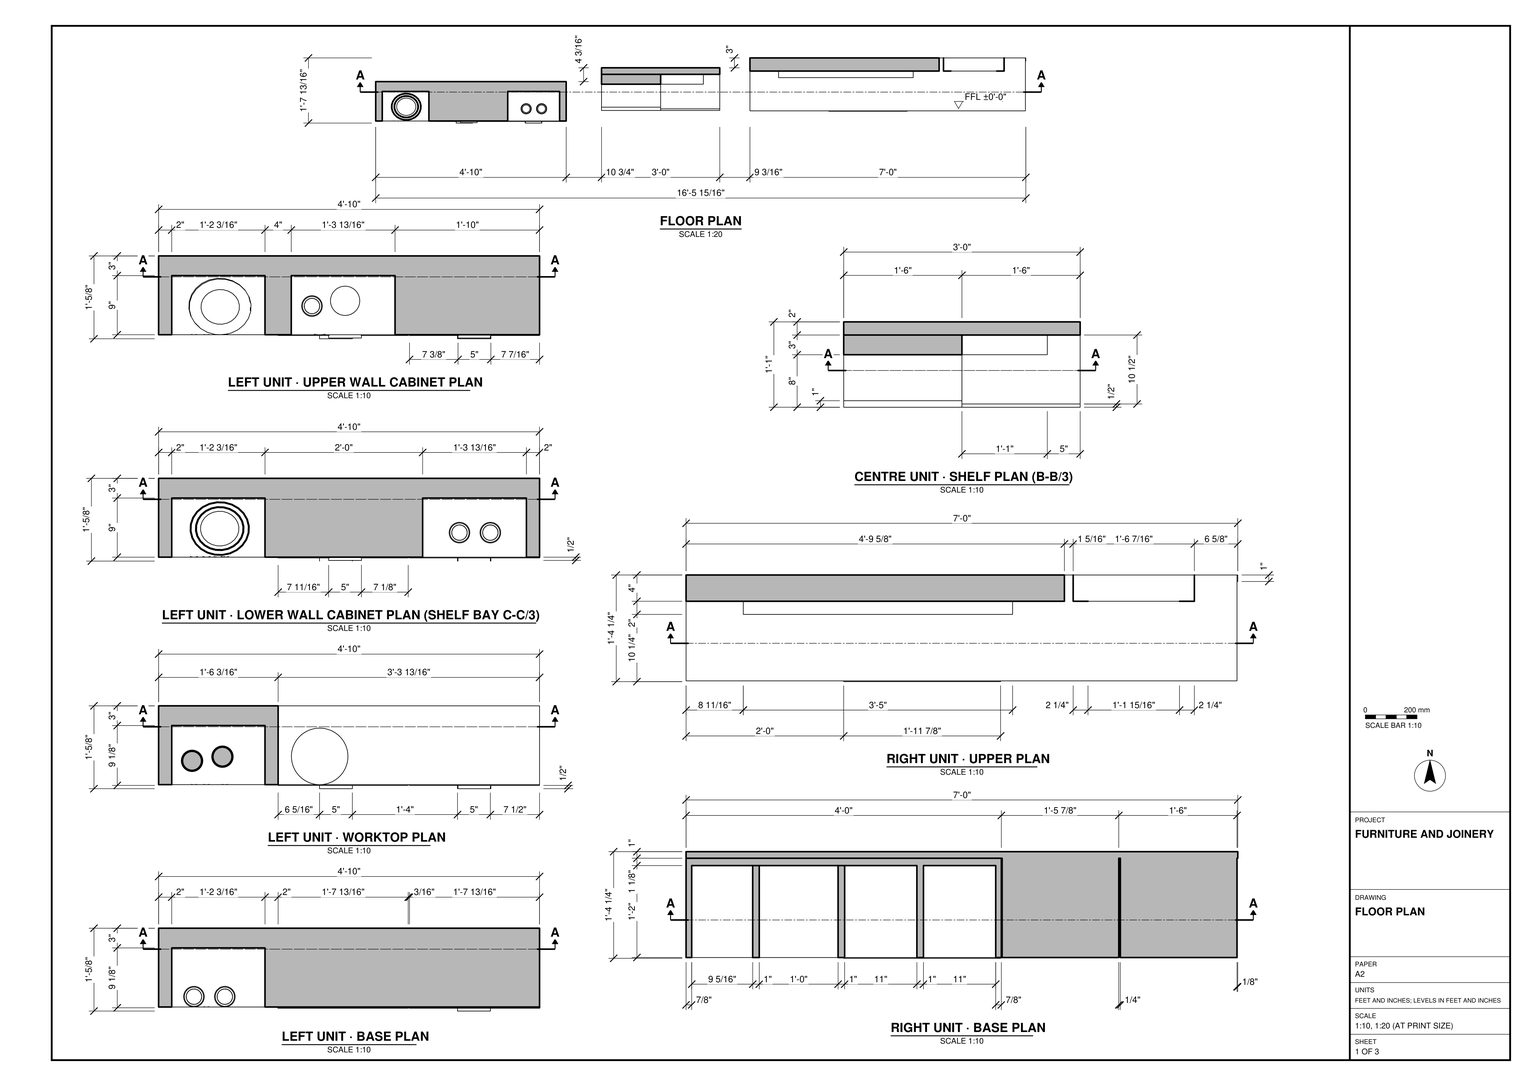
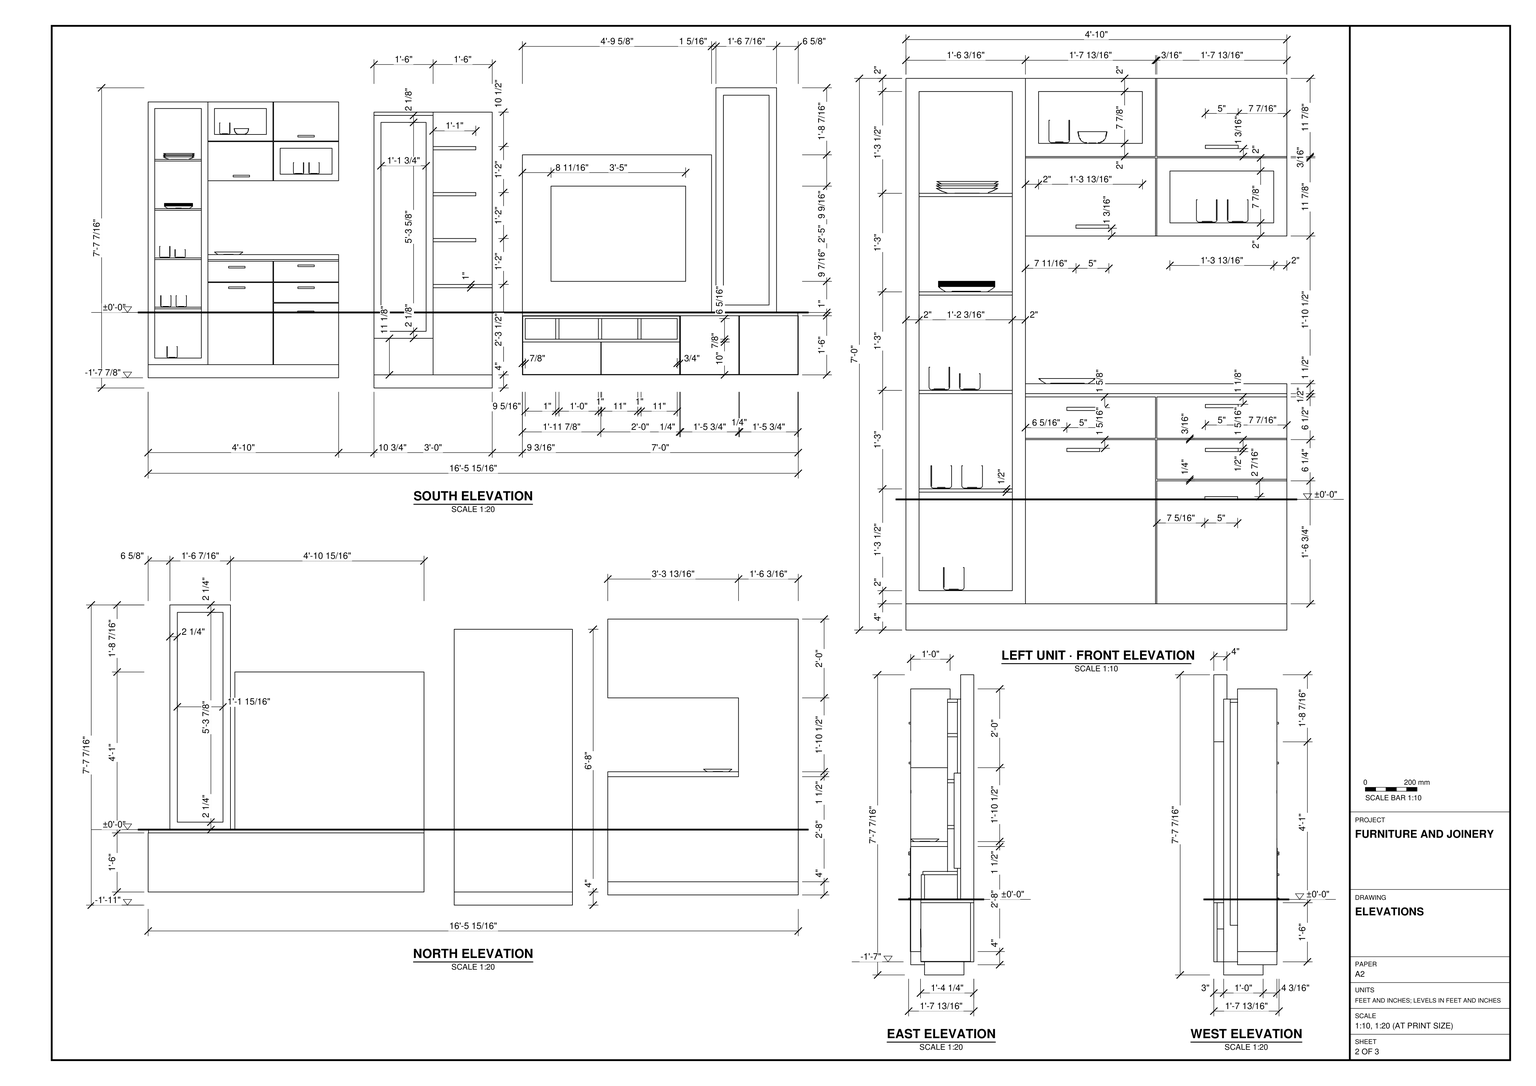
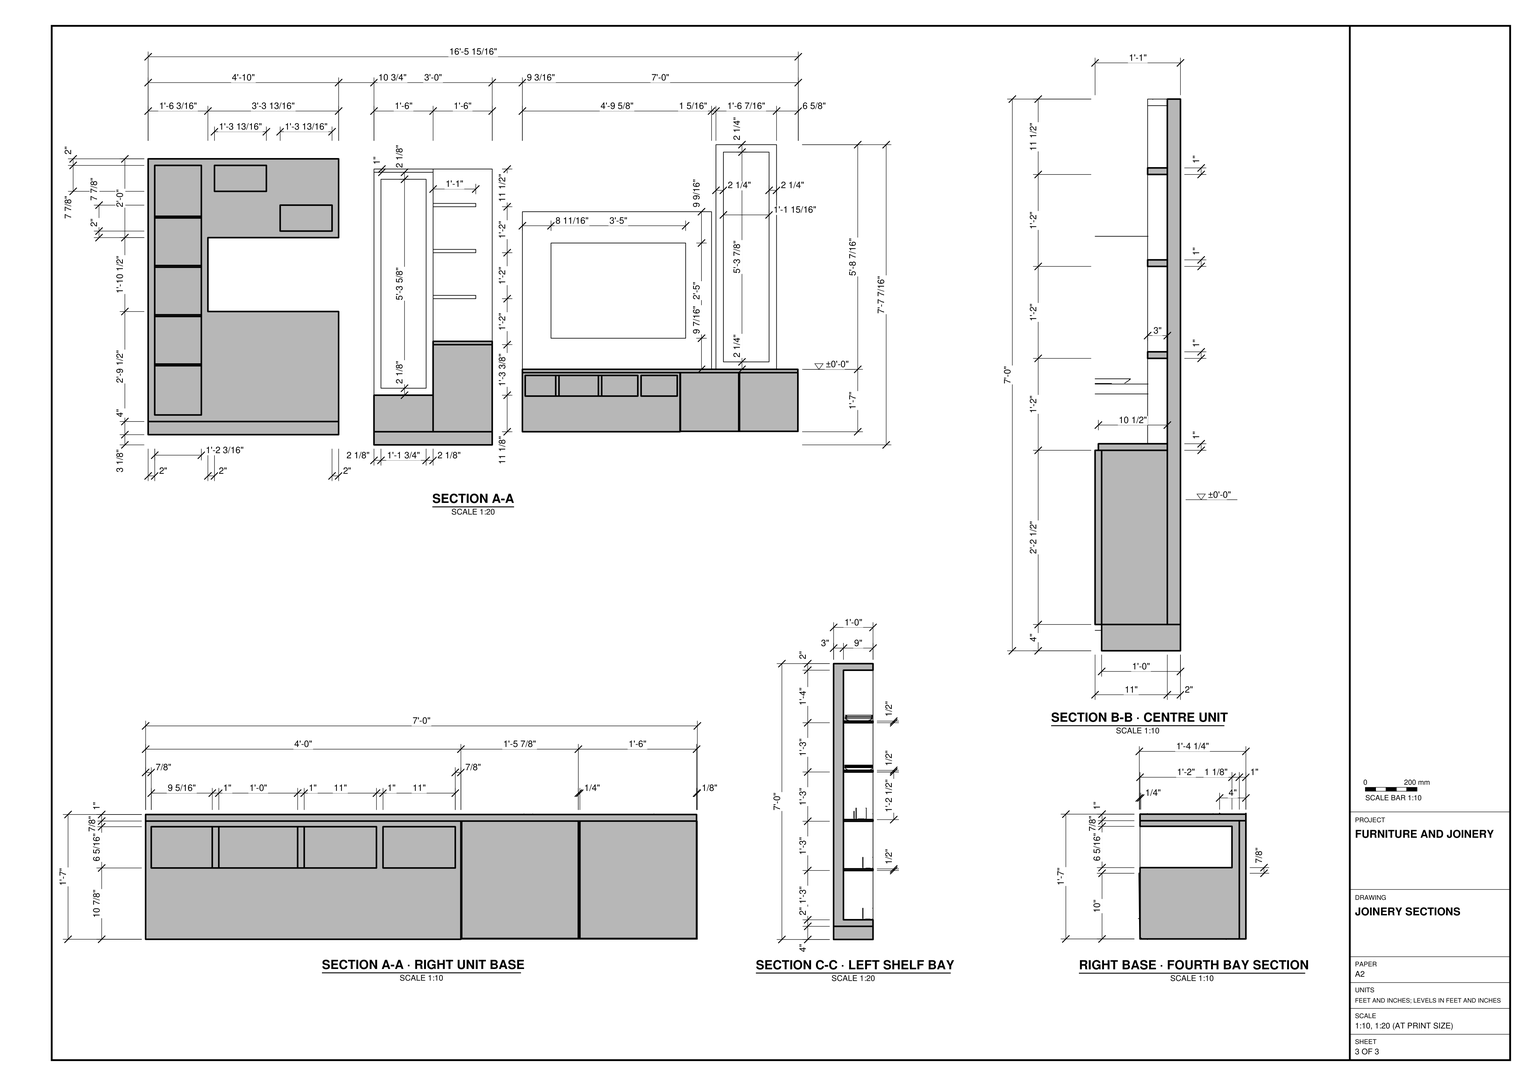
Build the joinery assembly in SketchUp from task_files/diagram_01.pdf. Work in feet and inches, with the finished-floor reference at ±0'-0". The assembly measures 16'-5 15/16" across, 1'-7 13/16" in overall depth and 7'-7 7/16" in overall height. Use the floor plan to set the gaps and front-to-back offsets between the units. Use section A-A to set their bases and tops relative to the reference level; the bases do not all sit at the same height.

On the left, build a full-height open shelf bay beside a worktop with storage below and wall cabinets above. Follow the front elevation for the drawer and cupboard divisions, pulls and open display compartments. In the centre unit, place the tall framed panel on the left and the projecting shelves on the right. On the right unit, build the long low cabinet with a row of shallow open compartments at its left end. Above it, model the wide rectangular panel and the taller, narrower framed panel. Use the detail plans and sections to give the backs, sides, shelves, plinths and fronts their drawn thicknesses and recesses.

Place dishes and cups in the left unit as shown. Decor and loose items may be any suitable library components. Keep each joinery piece in a separate group or component and use components for repeated parts. Save one SketchUp model as output_files/three_part_display_and_storage_unit.skp.

# SketchUp Ruby script. Lengths in inches.
U = 1.inch
M = Sketchup.active_model
def pt(a) = Geom::Point3d.new(a.map { |v| v * U })
def face(e, loops, mat)
  f = e.add_face(loops[0].map { |a| pt(a) })
  loops[1..].each { |l| e.add_face(l.map { |a| pt(a) }).erase! }
  f.material = f.back_material = mat if mat
  f
end
# faces: each face lists its corners as indices into pts; further lists are holes
def faces(e, pts, list, mat = nil) = list.each { |f| face(e, (f[0].is_a?(Array) ? f : [f]).map { |l| l.map { |i| pts[i] } }, mat) }
# xy, xz, yz: faces in a plane at the given z, y or x. An outline is a flat list of corners, or four numbers for a rectangle; further outlines are holes
def ring(l) = l.size == 4 ? [[l[0], l[1]], [l[2], l[1]], [l[2], l[3]], [l[0], l[3]]] : l.each_slice(2).to_a
def flat(e, list, mat, &to3) = list.each { |f| face(e, (f[0].is_a?(Array) ? f : [f]).map { |l| ring(l).map { |u, v| to3.(u, v) } }, mat) }
def xy(e, z, list, mat = nil) = flat(e, list, mat) { |x, y| [x, y, z] }
def xz(e, y, list, mat = nil) = flat(e, list, mat) { |x, z| [x, y, z] }
def yz(e, x, list, mat = nil) = flat(e, list, mat) { |y, z| [x, y, z] }
def lines(e, pts, list) = list.each { |a, b| e.add_line(pt(pts[a]), pt(pts[b])) }
# prism: a flat outline (further loops are holes) pulled along v
def prism(e, loops, v, mat = nil)
  f = face(e, loops, mat); d = Geom::Vector3d.new(v.map { |x| x * U })
  f.pushpull(f.normal.samedirection?(d) ? d.length : -d.length)
end
def box(e, o, s, mat = nil) = prism(e, [[o, [o[0] + s[0], o[1], o[2]], [o[0] + s[0], o[1] + s[1], o[2]], [o[0], o[1] + s[1], o[2]]]], [0, 0, s[2]], mat)
def at(x, y, z, deg = 0) = Geom::Transformation.translation(pt([x, y, z])) * Geom::Transformation.rotation(ORIGIN, Z_AXIS, deg.degrees)
def axes(o, x, y, z) = Geom::Transformation.new([*x, 0, *y, 0, *z, 0, *pt(o).to_a, 1])
def part(name) = M.definitions.add(name)
# library, detail: a bought-in or finely detailed component or shape, given as its bounding box
def library(name, o, s) = part(name).tap { |d| box(d.entities, o, s) }
def detail(e, o, s) = box(e.add_group.entities, o, s)
def put(e, d, t, mat = nil) = e.add_instance(d, t).tap { |i| i.material = mat if mat }
def group(e, t, mat = nil) = e.add_group.tap { |g| g.transformation = t; g.material = mat if mat }.entities
root = M.entities
M.materials.add("[Suede Dark Gray]").color = [85, 85, 85]
M.materials.add("[Wood Cherry Original]").color = [152, 86, 42]
M.materials.add("[Wood Floor Parquet]").color = [145, 89, 39]
M.materials.add("[Wood Veneer 01]").color = [120, 70, 37]
c1 = library("Cup (heat up)",[-27.01,0,-31.5],[48.56,5.94,71.64])
c2 = library("plates",[-46.18,-12,0],[25.68,8.61,38.39])
c3 = library("plates\#1",[10.82,85.4,0],[80.06,80.43,16.52])
c4 = part("Group\#8")
box(c4.entities,[0,0,0],[5,0.5,0.5])
c5 = part("Group\#3")
box(c5.entities,[0,0,0],[14.2,9,0.5])
c6 = part("Group\#4")
put(c6.entities,c5,at(0,0,0))
c7 = part("Group\#26")
g1 = group(c7.entities,at(0,0,0))
box(g1,[0,0,0],[13,1,3])
box(root,[38.2,0.5,8.72],[19.8,0.12,6.31])
box(root,[18.2,0.5,8.72],[19.8,0.12,6.31])
xy(root,-19.58,[[68.77,4.83,86.77,14.83],[86.77,4.83,104.77,14.83],[68.77,14.83,104.77,16.83]])
xy(root,-16.47,[[18.2,0.5,38,0.62],[38.2,0.5,58,0.62]])
xy(root,-8.45,[[68.77,4.83,86.77,11.83],[68.77,11.83,86.77,14.83]])
xy(root,2.25,[[38.2,0.5,58,0.62]])
xy(root,2.49,[[38.2,0.5,58,0.62]])
xy(root,6.94,[[86.77,4.83,104.77,14.83]])
xy(root,8.52,[[18.2,0.5,38,0.62],[38.2,0.5,58,0.62]])
xy(root,60.42,[[68.77,14.83,104.77,16.83]])
xz(root,0.5,[[18.2,-16.47,38,8.52],[38.2,-16.47,58,2.25],[38.2,2.49,58,8.52]],"[Wood Veneer 01]")
xz(root,0.62,[[18.2,-16.47,38,8.52],[38.2,-16.47,58,2.25],[38.2,2.49,58,8.52]])
xz(root,4.83,[[68.77,-19.58,86.77,-8.45]])
xz(root,11.83,[[[68.77,-8.45,86.77,59.42],[70.89,-6.33,84.65,57.3]],[70.89,-6.33,84.65,57.3]])
xz(root,14.83,[[86.77,-19.58,104.77,6.94],[68.77,-8.45,86.77,-8.45,86.77,6.94,104.77,6.94,104.77,60.42,68.77,60.42]])
xz(root,16.83,[[68.77,-19.58,104.77,60.42]])
yz(root,18.2,[[0.5,-16.47,0.62,8.52]])
yz(root,38,[[0.5,-16.47,0.62,8.52]])
yz(root,38.2,[[0.5,-16.47,0.62,2.25],[0.5,2.49,0.62,8.52]])
yz(root,58,[[0.5,-16.47,0.62,2.25],[0.5,2.49,0.62,8.52]])
yz(root,68.77,[[4.83,-19.58,4.83,-8.45,14.83,-8.45,14.83,60.42,16.83,60.42,16.83,-19.58]])
yz(root,86.77,[[4.83,-19.58,14.83,-8.45],[4.83,-8.45,11.83,6.94],[11.83,-8.45,14.83,6.94]])
yz(root,104.77,[[4.83,-19.58,14.83,6.94],[14.83,-19.58,16.83,60.42]])
put(root,c1,at(30.53,0.62,17.03))
put(root,c2,at(51.12,12.62,17.03))
put(root,c3,axes([3.33,-8.5,46.03],[0.11812,0,0],[0,0.10673,0],[0,0,0.10958]))
put(root,c4,at(45.59,0.12,52.85))
put(root,c4,at(25.89,0.12,40.71))
g2 = group(root,at(0,0.62,-20.47))
xy(g2,0,[[0,0,58,12]])
xy(g2,4,[[0,0,58,12]])
xy(g2,6,[[2,0,16.2,9]],"[Wood Cherry Original]")
xy(g2,37.5,[[18.2,0,58,12]],"[Suede Dark Gray]")
xy(g2,60,[[18.2,0,58,12]])
xy(g2,62,[[40.2,0,56,9]],"[Wood Veneer 01]")
xy(g2,69.9,[[40.2,0,56,9]])
xy(g2,74.1,[[20.2,0,36,9]],"[Wood Veneer 01]")
xy(g2,82,[[2,0,16.2,9]])
xy(g2,82,[[20.2,0,36,9]],"[Wood Veneer 01]")
xy(g2,84,[[0,0,58,12]])
xz(g2,0,[[0,0,58,4],[[0,4,18.2,84],[2,6,16.2,82]],[18.2,60,38,71.9],[[38.2,60,58,71.9],[40.2,62,56,69.9]],[[18.2,72.1,38,84],[20.2,74.1,36,82]],
  [38.2,72.1,58,84]])
xz(g2,0,[[18.2,36,58,37.5]],"[Suede Dark Gray]")
xz(g2,0,[[38,60,38.2,60,38.2,71.9,58,71.9,58,72.1,38.2,72.1,38.2,84,38,84,38,72.1,18.2,72.1,18.2,71.9,38,71.9]],"[Wood Cherry Original]")
xz(g2,0,[[18.2,4,58,36]],"[Wood Floor Parquet]")
xz(g2,9,[[2,6,16.2,82]],"[Wood Cherry Original]")
xz(g2,9,[[40.2,62,56,69.9],[20.2,74.1,36,82]],"[Wood Veneer 01]")
xz(g2,12,[[0,0,58,4],[0,4,0,84,58,84,58,60,18.2,60,18.2,36,58,36,58,4]])
xz(g2,12,[[18.2,36,58,37.5]],"[Suede Dark Gray]")
yz(g2,0,[[0,0,12,4],[0,4,12,84]])
yz(g2,2,[[0,6,9,82]],"[Wood Veneer 01]")
yz(g2,16.2,[[0,6,9,82]],"[Wood Veneer 01]")
yz(g2,18.2,[[0,37.5,12,60]])
yz(g2,20.2,[[0,74.1,9,82]],"[Wood Veneer 01]")
yz(g2,36,[[0,74.1,9,82]],"[Wood Veneer 01]")
yz(g2,40.2,[[0,62,9,69.9]],"[Wood Veneer 01]")
yz(g2,56,[[0,62,9,69.9]],"[Wood Veneer 01]")
yz(g2,58,[[0,0,12,4],[0,4,12,36],[0,60,12,84]])
yz(g2,58,[[0,36,12,37.5]],"[Suede Dark Gray]")
p = [[38,0,35.5],[18.2,0,35.5],[58,0,35.5],[38.2,0,35.5]]
lines(g2,p,[[0,1],[2,3]])
g3 = group(g2,at(2,0,21))
put(g3,c5,at(0,0,0))
put(g2,c6,at(2,0,36))
put(g2,c6,at(2,0,51))
put(g2,c6,at(2,0,66))
put(root,c4,at(45.59,0,6.7))
put(root,c4,at(45.59,0,13.38))
put(root,c4,at(45.51,0,-0.65))
put(root,c4,at(24.5,0,12.95))
put(root,c4,at(24.5,0,6.7))
g4 = group(root,at(68.77,4.83,-23.58))
g5 = group(g4,at(0,0,0))
box(g5,[0,0,0],[36,12,4])
g6 = group(root,at(68.77,4.83,-8.45))
box(g6,[0,7,0],[18,3,68.875])
g7 = group(root,at(68.77,11.83,60.42))
g8 = group(g7,at(0,0,-1))
box(g8,[0,0,0],[18,3,1])
g9 = group(root,at(68.77,4.83,-19.58),"[Wood Veneer 01]")
box(g9,[0,-1,0],[18,1,11.125])
g10 = group(root,at(42.76,-61.98,6.94))
g11 = group(g10,at(44,66.8125,0))
box(g11,[0,-0.5,0],[18,10.5,1])
g12 = group(root,at(86.77,4.83,-19.58),"[Wood Veneer 01]")
prism(g12,[[[18,0,0],[0,0,0],[0,0,11.125],[0,0,26.52],[18,0,26.52]]],[0,-1,0])
put(root,c7,axes([86.77,14.83,20.94],[1,0,0],[0,0,1],[0,-1,0]),"[Wood Veneer 01]")
put(root,c7,axes([86.77,14.83,34.94],[1,0,0],[0,0,1],[0,-1,0]),"[Wood Veneer 01]")
put(root,c7,axes([86.77,14.83,48.94],[1,0,0],[0,0,1],[0,-1,0]),"[Wood Veneer 01]")
g13 = group(root,at(113.96,3.83,-19.58))
xy(g13,0,[[0,15,84,16]])
xy(g13,0.12,[[24,-0.12,24.12,0],[24.12,-0.12,47.88,0],[48.12,-0.12,65.88,15],[66.12,-0.12,83.88,15]])
xy(g13,10,[[24,-0.24,47.88,-0.12]])
xy(g13,18,[[48.12,-0.12,65.88,15],[66.12,-0.12,83.88,15],[0,15,84,16]])
xz(g13,-0.12,[[48.12,0.12,65.88,18],[66.12,0.12,83.88,18]])
xz(g13,15,[[0,0,84,0,84,18,83.88,18,83.88,0.12,66.12,0.12,66.12,18,65.88,18,65.88,0.12,48.12,0.12,48.12,18,0,18]])
xz(g13,16,[[0,0,84,18]])
yz(g13,0,[[15,0,16,18]])
yz(g13,24,[[-0.12,0.12,-0.24,10,-0.12,10,0,0.12]])
yz(g13,47.88,[[-0.12,0.12,0,0.12,-0.12,10,-0.24,10]])
yz(g13,48.12,[[-0.12,0.12,15,18]])
yz(g13,65.88,[[-0.12,0.12,15,18]])
yz(g13,66.12,[[-0.12,0.12,15,18]])
yz(g13,83.88,[[-0.12,0.12,15,18]])
yz(g13,84,[[15,0,16,18]])
p = [[24.12,-0.12,0.12],[47.88,-0.12,0.12],[47.88,-0.24,10],[24,-0.24,10],[24,-0.12,0.12],[47.88,0,0.12],
  [47.88,0,17.88],[24.12,0,17.88],[0.12,0,0.12],[23.88,0,0.12],[23.88,0,17.88],[0.12,0,17.88]]
faces(g13,p,[[0,1,2,3,4]])
lines(g13,p,[[5,6],[6,7],[8,9],[10,11],[11,8]])
g14 = group(root,at(122.67,13.83,8.89))
xz(g14,0,[[0,0,41,29]])
g15 = group(root,at(113.96,3.71,-19.58))
xy(g15,0,[[23.88,0,48,15.12],[0,0.12,23.88,15.12]])
xy(g15,0.12,[[0.12,0,23.88,0.12]])
xy(g15,10,[[0,0,0.12,0.12],[0.12,0,23.88,0.12]])
xy(g15,10.86,[[0.86,0,11.14,14],[11.14,0,24.14,14],[24.14,0,35.14,14],[36.14,0,47.14,14]],"[Wood Veneer 01]")
xy(g15,17.14,[[0.86,0,11.14,14],[11.14,0,24.14,14],[24.14,0,35.14,14],[36.14,0,47.14,14]])
xy(g15,18,[[0,0,48,15.12],[48,0,48,15.12,0,15.12,0,16.12,83.88,16.12,83.88,0]])
xy(g15,19,[[0,12.12,57.6,16.12],[58.9375,12.12,77.39,16.12]])
xy(g15,19,[[0,0,83.88,0,83.88,16.12,77.39,16.12,77.39,12.12,58.9375,12.12,58.9375,16.12,57.6,16.12,57.6,12.12,0,12.12]],"[Wood Veneer 01]")
xy(g15,28.46,[[8.71,10.12,49.71,12.12]])
xy(g15,57.46,[[8.71,10.12,49.71,12.12]])
xy(g15,67,[[0,12.12,57.6,16.12]])
xy(g15,87.42,[[58.9375,12.12,77.39,16.12]])
xz(g15,0,[[0.12,0.12,23.88,10]])
xz(g15,0,[[[23.88,0,48,0,48,18,0,18,0,10,23.88,10],[0.86,10.86,47.14,17.14]],[10.14,10.86,11.14,17.14],[23.14,10.86,24.14,17.14],[35.14,10.86,36.14,17.14],[0,18,83.88,19]],"[Wood Veneer 01]")
xz(g15,0.12,[[0,0,23.88,0,23.88,0.12,0.12,0.12,0.12,10,0,10],[0.12,0.12,23.88,10]])
xz(g15,12.12,[[[0,19,57.6,67],[8.71,28.46,49.71,57.46]],[[58.9375,19,77.39,87.42],[61.21,21.27,75.12,85.15]]])
xz(g15,14,[[0.86,10.86,11.14,17.14],[11.14,10.86,24.14,17.14],[24.14,10.86,35.14,17.14],[36.14,10.86,47.14,17.14]],"[Wood Veneer 01]")
xz(g15,15.12,[[0,0,48,18]])
xz(g15,16.12,[[0,19,57.6,67]])
xz(g15,16.12,[[0,18,83.88,19]],"[Wood Veneer 01]")
yz(g15,0,[[0.12,0,15.12,10],[0,10,15.12,18],[12.12,19,16.12,67]])
yz(g15,0,[[0,18,16.12,19]],"[Wood Veneer 01]")
yz(g15,0.12,[[0,0.12,0.12,10]])
yz(g15,0.86,[[0,10.86,14,17.14]],"[Wood Veneer 01]")
yz(g15,8.71,[[10.12,28.46,12.12,57.46]])
yz(g15,10.14,[[0,10.86,14,17.14]],"[Wood Veneer 01]")
yz(g15,11.14,[[0,10.86,14,17.14]],"[Wood Veneer 01]")
yz(g15,23.14,[[0,10.86,14,17.14]],"[Wood Veneer 01]")
yz(g15,23.88,[[0,0,0.12,0.12],[0,0.12,0.12,10]])
yz(g15,24.14,[[0,10.86,14,17.14]],"[Wood Veneer 01]")
yz(g15,35.14,[[0,10.86,14,17.14]],"[Wood Veneer 01]")
yz(g15,36.14,[[0,10.86,14,17.14]],"[Wood Veneer 01]")
yz(g15,47.14,[[0,10.86,14,17.14]],"[Wood Veneer 01]")
yz(g15,48,[[0,0,15.12,18]])
yz(g15,49.71,[[10.12,28.46,12.12,57.46]])
yz(g15,57.6,[[12.12,19,16.12,67]])
yz(g15,58.9375,[[12.12,19,16.12,87.42]])
yz(g15,77.39,[[12.12,19,16.12,87.42]])
yz(g15,83.88,[[0,18,16.12,19]],"[Wood Veneer 01]")
